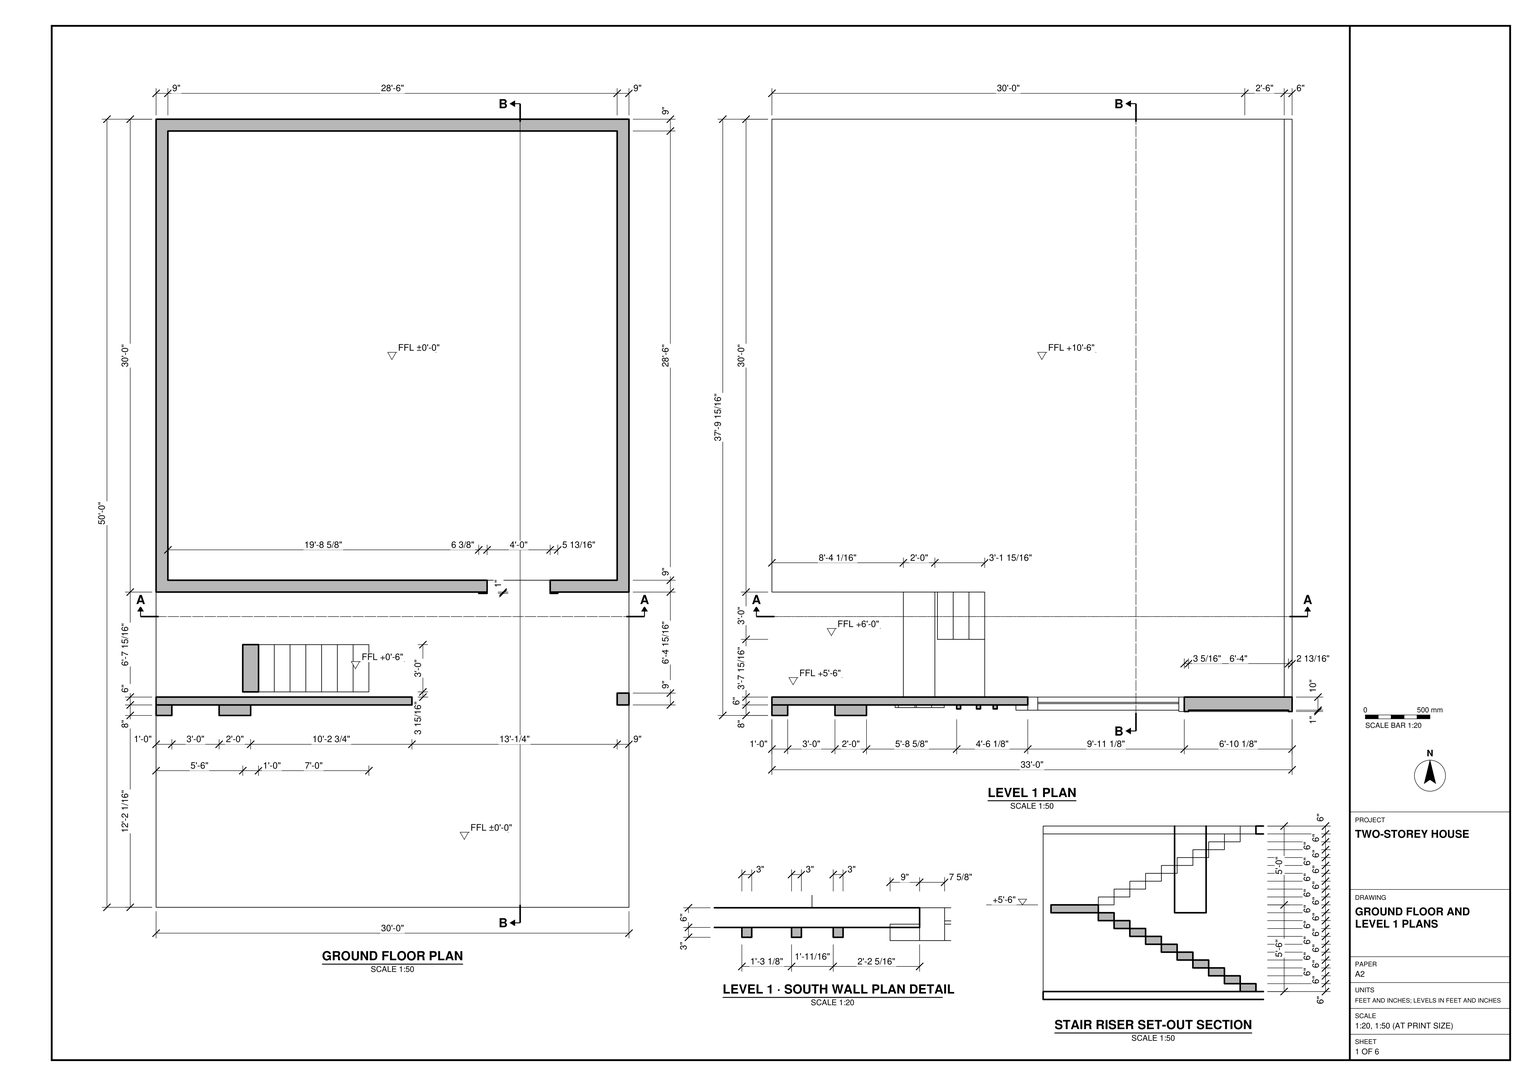
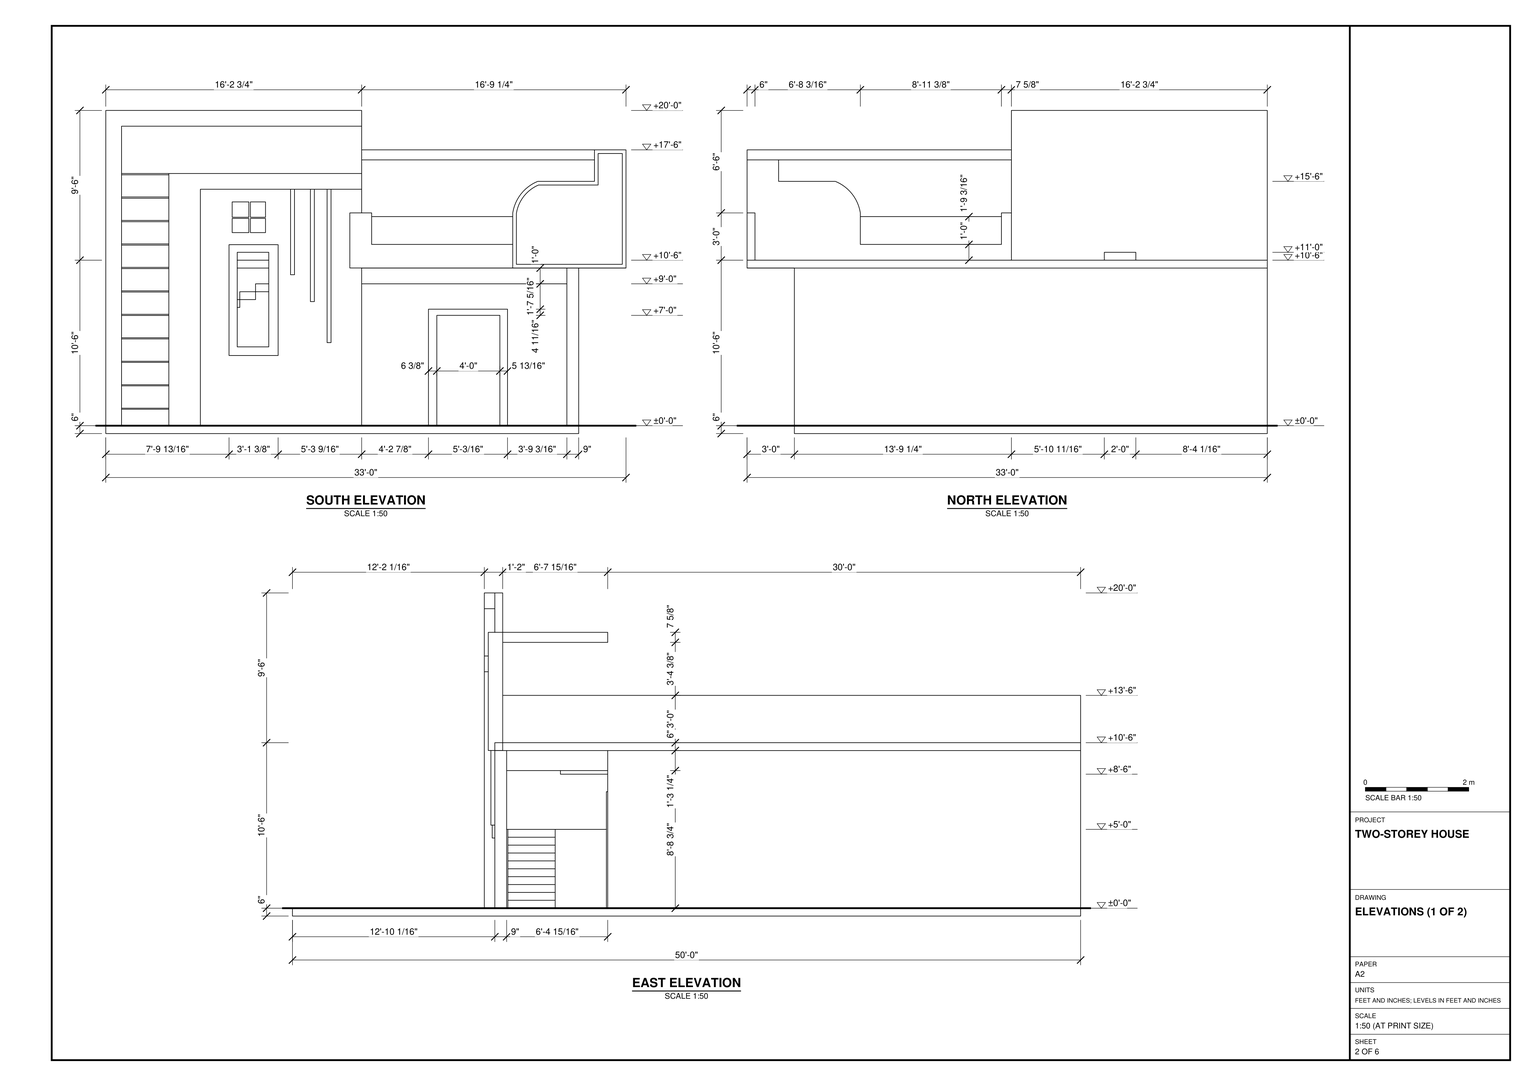
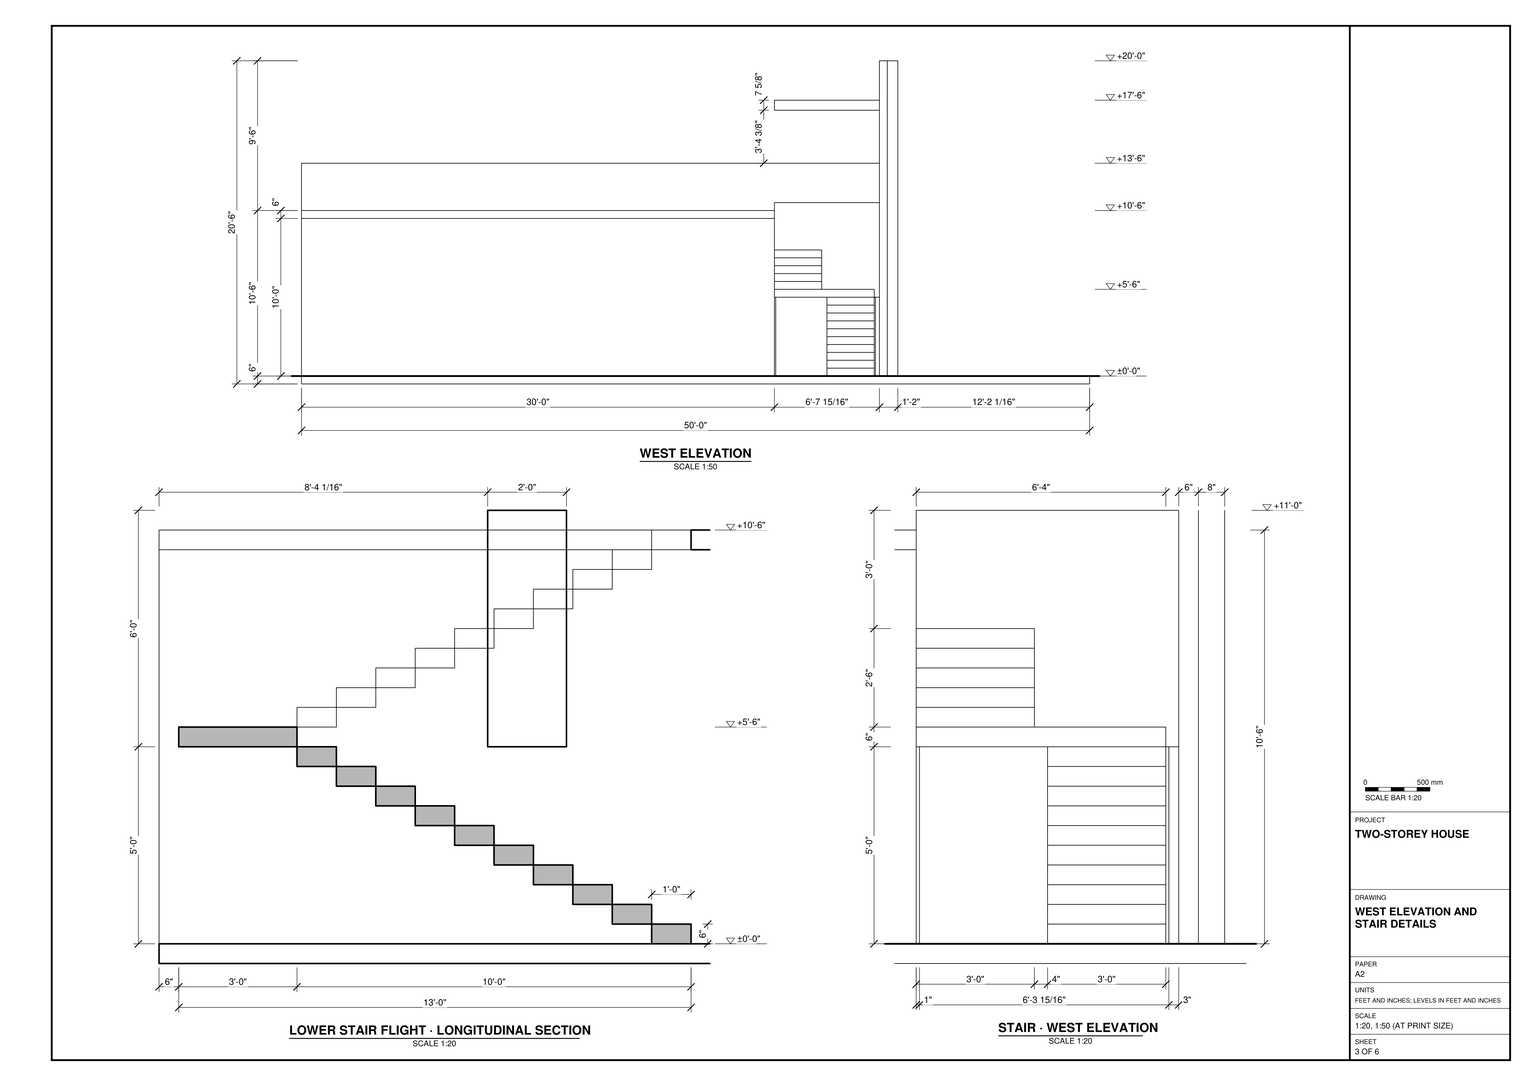
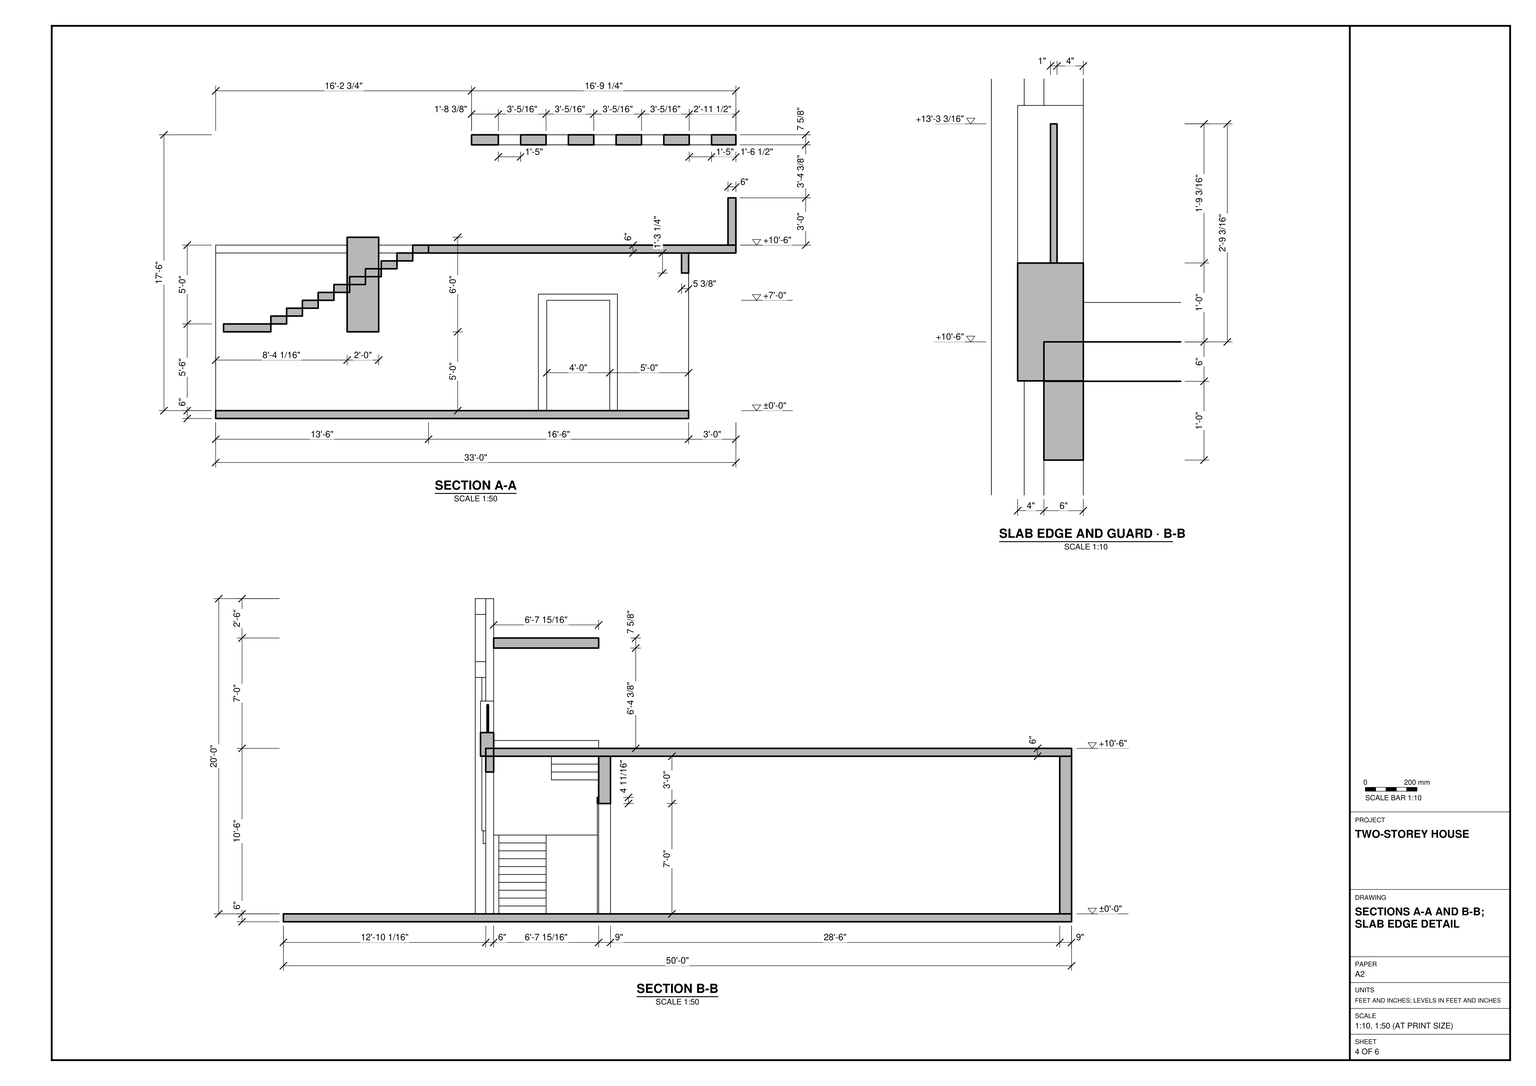
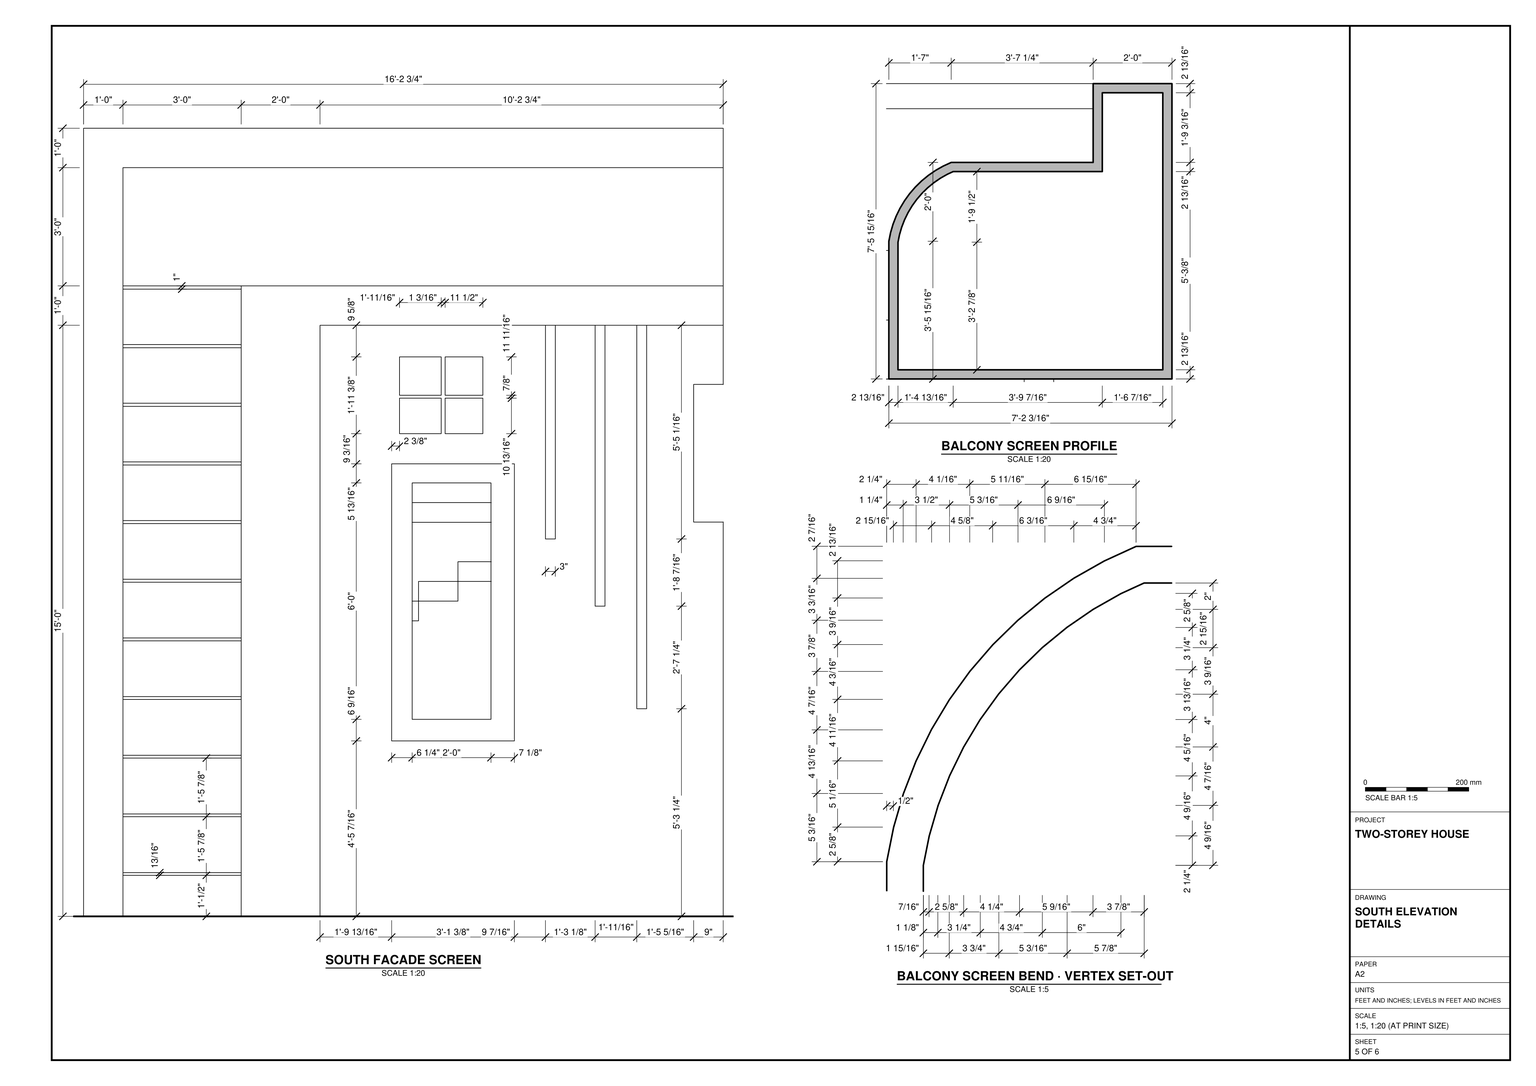
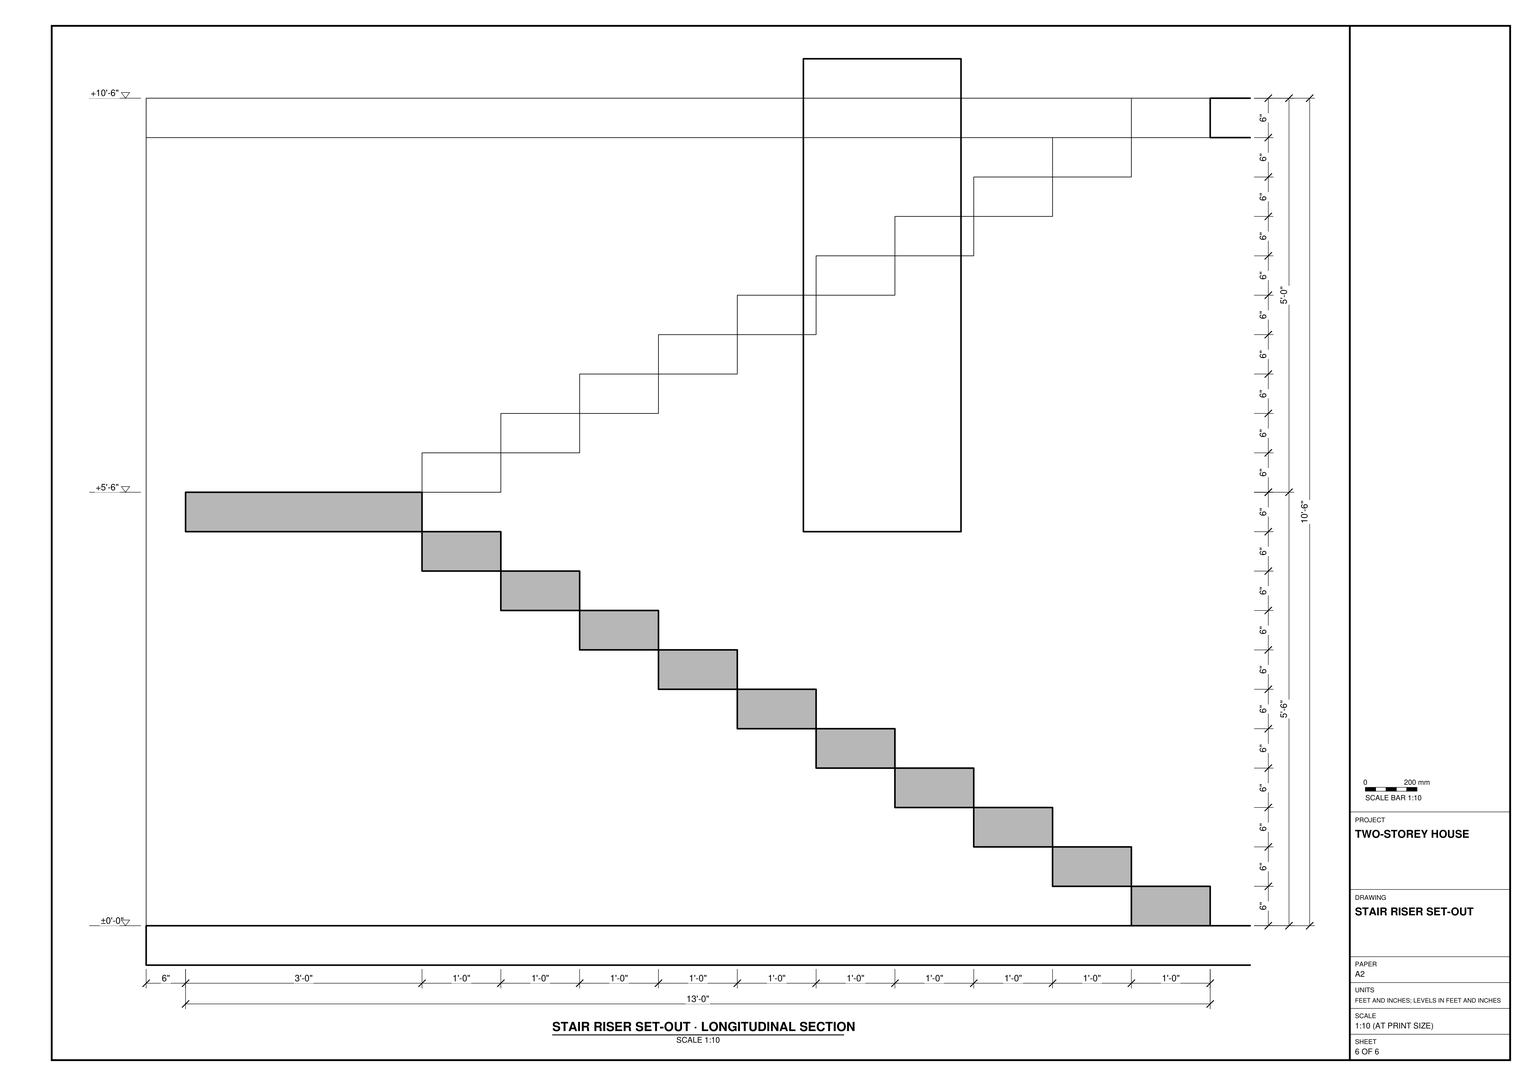
Build the house shown in task_files/diagram_01.pdf in SketchUp. Work in feet and inches. The overall model is 33'-0" wide east to west, 50'-0" deep north to south and 20'-6" high from the underside of the base slab to the top of the south screen. Set the finished floor levels at ±0'-0" and +10'-6".

Place the 30'-0" square ground-floor enclosure at the north end of the base slab. Use the drawn 9" wall thickness and leave the doorway toward the east end of its south wall. Model the flat roof slab as the Level 1 terrace, including its projection beyond the enclosure, its edge walls and the opening for the stair. Between the enclosure and the south screen, model the stair as two parallel flights that reverse direction at the +5'-6" landing. Follow the stair sections for the tread profile and the open space beneath the flights.

Use the elevations to shape the south screen on both sides of the entrance. Include the horizontal divisions at the left, the framed rectangular detail with a divided square above it, the narrow vertical strips and the curved shoulder of the upper panel at the right.

Keep walls, slabs and roof elements in separate groups or components, and do the same for each furniture or joinery piece shown. Use components for repeated parts. Any decor or loose items shown may be represented by suitable library components. Save one SketchUp model as output_files/two_storey_house_with_a_return_stair_and_south_screen.skp.

# SketchUp Ruby script. Lengths in inches.
U = 1.inch
M = Sketchup.active_model
def pt(a) = Geom::Point3d.new(a.map { |v| v * U })
def face(e, loops, mat)
  f = e.add_face(loops[0].map { |a| pt(a) })
  loops[1..].each { |l| e.add_face(l.map { |a| pt(a) }).erase! }
  f.material = f.back_material = mat if mat
  f
end
# faces: each face lists its corners as indices into pts; further lists are holes
def faces(e, pts, list, mat = nil) = list.each { |f| face(e, (f[0].is_a?(Array) ? f : [f]).map { |l| l.map { |i| pts[i] } }, mat) }
# xy, xz, yz: faces in a plane at the given z, y or x. An outline is a flat list of corners, or four numbers for a rectangle; further outlines are holes
def ring(l) = l.size == 4 ? [[l[0], l[1]], [l[2], l[1]], [l[2], l[3]], [l[0], l[3]]] : l.each_slice(2).to_a
def flat(e, list, mat, &to3) = list.each { |f| face(e, (f[0].is_a?(Array) ? f : [f]).map { |l| ring(l).map { |u, v| to3.(u, v) } }, mat) }
def xy(e, z, list, mat = nil) = flat(e, list, mat) { |x, y| [x, y, z] }
def xz(e, y, list, mat = nil) = flat(e, list, mat) { |x, z| [x, y, z] }
def yz(e, x, list, mat = nil) = flat(e, list, mat) { |y, z| [x, y, z] }
def lines(e, pts, list) = list.each { |a, b| e.add_line(pt(pts[a]), pt(pts[b])) }
# prism: a flat outline (further loops are holes) pulled along v
def prism(e, loops, v, mat = nil)
  f = face(e, loops, mat); d = Geom::Vector3d.new(v.map { |x| x * U })
  f.pushpull(f.normal.samedirection?(d) ? d.length : -d.length)
end
def box(e, o, s, mat = nil) = prism(e, [[o, [o[0] + s[0], o[1], o[2]], [o[0] + s[0], o[1] + s[1], o[2]], [o[0], o[1] + s[1], o[2]]]], [0, 0, s[2]], mat)
def at(x, y, z, deg = 0) = Geom::Transformation.translation(pt([x, y, z])) * Geom::Transformation.rotation(ORIGIN, Z_AXIS, deg.degrees)
def axes(o, x, y, z) = Geom::Transformation.new([*x, 0, *y, 0, *z, 0, *pt(o).to_a, 1])
def part(name) = M.definitions.add(name)
# library, detail: a bought-in or finely detailed component or shape, given as its bounding box
def library(name, o, s) = part(name).tap { |d| box(d.entities, o, s) }
def detail(e, o, s) = box(e.add_group.entities, o, s)
def put(e, d, t, mat = nil) = e.add_instance(d, t).tap { |i| i.material = mat if mat }
def group(e, t, mat = nil) = e.add_group.tap { |g| g.transformation = t; g.material = mat if mat }.entities
root = M.entities
M.materials.add("[Formica Blue]").color = [71, 97, 152]
M.materials.add("[Terrazzo Light Blue]").color = [196, 214, 227]
M.materials.add("[Translucent Glass Gray]").color = [128, 128, 128]
M.materials["[Translucent Glass Gray]"].alpha = 0.5
M.materials.add("[Wood OSB]").color = [240, 195, 122]
c1 = part("Stair tread")
box(c1.entities,[0,0,0],[12,36,6])
c2 = part("Stair landing")
box(c2.entities,[0,0,0],[36,76,6])
prism(root,[[[252,240,90],[252,240,6],[245.625,240,6],[245.625,240,94.6875],[305.81,240,94.6875],[305.81,240,6],[300,240,6],[300,240,90]]],[0,-1,0])
xy(root,6,[[0,146.0625,12,154.0625],[48,146.0625,72,154.0625]])
xy(root,59.43,[[93.8125,152.0625,131.1875,154.0625]])
xy(root,66,[[100.0625,152.0625,124.0625,240]])
xy(root,69.23,[[168.46,151.0625,171.46,154.0625]])
xy(root,100.46,[[155.77,151.0625,158.77,154.0625]])
xy(root,120.93,[[140.65,151.0625,143.65,154.0625]])
xy(root,132,[[390,160.0625,396,600]])
xy(root,138,[[100.0625,152.0625,124.0625,240]])
xy(root,143.8,[[93.8125,152.0625,100.0625,154.0625],[100.0625,152.0625,131.1875,154.0625]])
xy(root,144,[[202.39,155.0625,309.79,156.0625]])
xy(root,152.99,[[96.21,152.0625,108.9,154.0625],[110.1,152.0625,121.59,154.0625]])
xy(root,163.8,[[96.21,152.0625,108.9,154.0625],[110.1,152.0625,121.59,154.0625]])
xy(root,164.68,[[96.21,152.0625,108.9,154.0625],[110.1,152.0625,121.59,154.0625]])
xy(root,165.1875,[[202.39,155.0625,309.79,156.0625]],"[Translucent Glass Gray]")
xy(root,168,[[390,160.0625,396,600]])
xy(root,176.37,[[96.21,152.0625,108.9,154.0625],[110.1,152.0625,121.59,154.0625]])
xy(root,186,[[72,146.0625,72,154.0625,140.65,154.0625,140.65,151.0625,143.65,151.0625,143.65,154.0625,155.77,154.0625,155.77,151.0625,158.77,151.0625,158.77,154.0625,168.46,154.0625,168.46,151.0625,171.46,151.0625,171.46,154.0625,194.77,154.0625,194.77,146.0625],[140.65,151.0625,143.65,154.0625],[155.77,151.0625,158.77,154.0625],[168.46,151.0625,171.46,154.0625]])
xy(root,198,[[48,146.0625,194.77,154.0625]],"[Terrazzo Light Blue]")
xy(root,234,[[12,146.0625,194.77,154.0625]])
xy(root,246,[[0,146.0625,194.77,154.0625]])
xz(root,146.0625,[[0,6,12,6,12,234,194.77,234,194.77,246,0,246],[48,6,72,6,72,186,194.77,186,194.77,198,48,198]],"[Terrazzo Light Blue]")
xz(root,151.0625,[[168.46,69.23,171.46,186],[155.77,100.46,158.77,186],[140.65,120.93,143.65,186]],"[Wood OSB]")
xz(root,152.0625,[[[93.8125,59.43,131.1875,143.8],[100.0625,66,124.0625,138]],[96.21,152.99,108.9,163.8],[110.1,152.99,121.59,163.8],[96.21,164.68,108.9,176.37],[110.1,164.68,121.59,176.37]],"[Wood OSB]")
xz(root,154.0625,[[0,6,0,246,194.77,246,194.77,234,12,234,12,6],[48,6,48,198,194.77,198,194.77,186,72,186,72,6],[[93.8125,59.43,131.1875,143.8],[100.0625,66,124.0625,138]],[168.46,69.23,171.46,186],[155.77,100.46,158.77,186],
  [140.65,120.93,143.65,186],[96.21,152.99,108.9,163.8],[110.1,152.99,121.59,163.8],[96.21,164.68,108.9,176.37],[110.1,164.68,121.59,176.37]])
xz(root,155.0625,[[202.39,144,309.79,165.1875]],"[Translucent Glass Gray]")
xz(root,156.0625,[[202.39,144,309.79,165.1875]],"[Translucent Glass Gray]")
xz(root,160.0625,[[390,132,396,168]])
xz(root,240,[[100.0625,66,124.0625,138]])
xz(root,600,[[390,132,396,168]])
yz(root,0,[[146.0625,6,154.0625,246]])
yz(root,12,[[146.0625,6,154.0625,234]],"[Terrazzo Light Blue]")
yz(root,48,[[146.0625,6,154.0625,198]])
yz(root,72,[[146.0625,6,154.0625,186]],"[Terrazzo Light Blue]")
yz(root,93.8125,[[152.0625,59.43,154.0625,143.8]])
yz(root,96.21,[[152.0625,152.99,154.0625,163.8],[152.0625,164.68,154.0625,176.37]])
yz(root,100.0625,[[152.0625,66,240,138]])
yz(root,108.9,[[152.0625,152.99,154.0625,163.8],[152.0625,164.68,154.0625,176.37]])
yz(root,110.1,[[152.0625,152.99,154.0625,163.8],[152.0625,164.68,154.0625,176.37]])
yz(root,121.59,[[152.0625,152.99,154.0625,163.8],[152.0625,164.68,154.0625,176.37]])
yz(root,124.0625,[[152.0625,66,240,138]])
yz(root,131.1875,[[152.0625,59.43,154.0625,143.8]])
yz(root,140.65,[[151.0625,120.93,154.0625,186]])
yz(root,143.65,[[151.0625,120.93,154.0625,186]])
yz(root,155.77,[[151.0625,100.46,154.0625,186]])
yz(root,158.77,[[151.0625,100.46,154.0625,186]])
yz(root,168.46,[[151.0625,69.23,154.0625,186]])
yz(root,171.46,[[151.0625,69.23,154.0625,186]])
yz(root,194.77,[[146.0625,186,154.0625,198],[146.0625,234,154.0625,246]])
yz(root,202.39,[[155.0625,144,156.0625,165.1875]])
yz(root,309.79,[[155.0625,144,156.0625,165.1875]])
yz(root,390,[[160.0625,132,600,168]])
yz(root,396,[[160.0625,132,600,168]],"[Terrazzo Light Blue]")
p = [[12,154.0625,198],[48,154.0625,198],[12,154.0625,180.13],[48,154.0625,180.13],[12,154.0625,162.26],[48,154.0625,162.26],
  [12,154.0625,144.39],[48,154.0625,144.39],[12,154.0625,126.52],[48,154.0625,126.52],[12,154.0625,108.66],[48,154.0625,108.66],
  [12,154.0625,90.79],[48,154.0625,90.79],[12,154.0625,72.92],[48,154.0625,72.92],[12,154.0625,55.05],[48,154.0625,55.05],
  [12,154.0625,37.18],[48,154.0625,37.18],[12,154.0625,19.3125],[48,154.0625,19.3125],[12,154.0625,197],[48,154.0625,197],
  [12,154.0625,179.15],[48,154.0625,179.15],[12,154.0625,161.3],[48,154.0625,161.3],[12,154.0625,143.45],[48,154.0625,143.45],
  [12,154.0625,125.6],[48,154.0625,125.6],[12,154.0625,107.75],[48,154.0625,107.75],[12,154.0625,89.9],[48,154.0625,89.9],
  [12,154.0625,72.05],[48,154.0625,72.05],[12,154.0625,54.2],[48,154.0625,54.2],[12,154.0625,36.35],[48,154.0625,36.35],
  [12,154.0625,18.5],[48,154.0625,18.5]]
lines(root,p,[[0,1],[2,3],[4,5],[6,7],[8,9],[10,11],[12,13],[14,15],[16,17],[18,19],[20,21],[22,23],
  [24,25],[26,27],[28,29],[30,31],[32,33],[34,35],[36,37],[38,39],[40,41],[42,43]])
put(root,c1,at(150,164,6))
put(root,c1,at(138,164,12))
put(root,c1,at(126,164,18))
put(root,c1,at(114,164,24))
put(root,c1,at(102,164,30))
put(root,c1,at(90,164,36))
put(root,c1,at(78,164,42))
put(root,c1,at(66,164,48))
put(root,c1,at(54,164,54))
put(root,c1,at(42,164,60))
put(root,c1,at(54,240,72,180))
put(root,c1,at(78,240,84,180))
put(root,c1,at(162,240,126,180))
put(root,c1,at(126,240,108,180))
put(root,c1,at(66,240,78,180))
put(root,c1,at(150,240,120,180))
put(root,c1,at(90,240,90,180))
put(root,c1,at(102,240,96,180))
put(root,c1,at(114,240,102,180))
put(root,c1,at(138,240,114,180))
put(root,c2,at(6,164,66))
g1 = group(root,at(0,240,0))
box(g1,[0,-240,0],[360,600,6])
g2 = group(root,at(0,240,126))
prism(g2,[[[0,0,0],[0,360,0],[396,360,0],[396,-85.9375,0],[194.77,-85.9375,0],[194.77,-79.9375,0],[162,-79.9375,0],[162,0,0]]],[0,0,6])
g3 = group(root,at(0,240,6),"[Terrazzo Light Blue]")
xy(g3,0,[[0,0,0,360,360,360,360,0,300,0,300,9,351,9,351,351,9,351,9,9,252,9,252,0],[9,9,351,351]])
xy(g3,84,[[252,0,300,9]])
xy(g3,120,[[[0,0,360,360],[9,9,351,351]]])
xz(g3,0,[[0,0,252,0,252,84,300,84,300,0,360,0,360,120,0,120]])
xz(g3,9,[[9,0,9,120,351,120,351,0,300,0,300,84,252,84,252,0]])
xz(g3,351,[[9,0,351,120]])
xz(g3,360,[[0,0,360,120]])
yz(g3,0,[[0,0,360,120]])
yz(g3,9,[[9,0,351,120]])
yz(g3,252,[[0,0,9,84]])
yz(g3,300,[[0,0,9,84]])
yz(g3,351,[[9,0,351,120]])
yz(g3,360,[[0,0,360,120]])
g4 = group(root,at(0,154.0625,6),"[Formica Blue]")
prism(g4,[[[194.77,6,0],[0,6,0],[0,6,240],[194.77,6,240]],[[100.0625,6,60],[124.0625,6,60],[124.0625,6,132],[100.0625,6,132]]],[0,-6,0])
g5 = group(root,at(351,154.0625,6),"[Terrazzo Light Blue]")
box(g5,[0,0,0],[9,9,120])
g6 = group(root,at(194.77,154.0625,114),"[Terrazzo Light Blue]")
box(g6,[0,0,0],[156.23,6,12])
g7 = group(root,at(354.625,163.0625,110.75),"[Terrazzo Light Blue]")
box(g7,[0,0,0],[5.375,76.9375,15.25])
g8 = group(root,at(185.77,150.0625,126.0625),"[Terrazzo Light Blue]")
xy(g8,0,[[124.02,-1,124.02,0,0,0,0,4,9,4,9,10,210.23,10,210.23,-1]])
xy(g8,2.79,[[126.8,-1,207.4375,0]])
xy(g8,17.9375,[[16.61,0,124.02,10]])
xy(g8,41.9375,[[0,0,9,5],[9,0,16.61,10]])
xy(g8,63.15,[[143.6,-1,189.01,0]])
xy(g8,65.9375,[[142.99,-1,186.23,10]])
xy(g8,87.15,[[189.01,-1,207.4375,0]])
xy(g8,89.9375,[[186.23,-1,210.23,10]])
xz(g8,-1,[[[124.02,0,210.23,0,210.23,89.9375,186.23,89.9375,186.23,65.9375,142.99,65.9375,140.57,64.83,138.25,63.51,136.06,62,134,60.3125,132.09,58.45,130.35,56.43,128.79,54.27,127.42,51.99,126.24,49.6,125.28,47.11,124.54,44.55,124.02,41.9375],[126.8,2.79,126.8,41.66,127.25,43.89,127.93,46.22,128.8,48.48,129.87,50.66,131.12,52.74,132.54,54.7,134.12,56.54,135.86,58.23,137.73,59.77,139.73,61.15,141.84,62.34,143.6,63.15,189.01,63.15,189.01,87.15,207.4375,87.15,207.4375,2.79]]],"[Wood OSB]")
xz(g8,0,[[0,0,124.02,0,124.02,17.9375,16.61,17.9375,16.61,41.9375,0,41.9375]])
xz(g8,0,[[126.8,2.79,207.4375,2.79,207.4375,87.15,189.01,87.15,189.01,63.15,143.6,63.15,141.84,62.34,139.73,61.15,137.73,59.77,135.86,58.23,134.12,56.54,132.54,54.7,131.12,52.74,129.87,50.66,128.8,48.48,127.93,46.22,127.25,43.89,126.8,41.66]],"[Formica Blue]")
xz(g8,4,[[0,0,9,5.9375]])
xz(g8,10,[[9,0,9,41.9375,16.61,41.9375,16.61,17.9375,124.02,17.9375,124.02,41.9375,124.54,44.55,125.28,47.11,126.24,49.6,127.42,51.99,128.79,54.27,130.35,56.43,132.09,58.45,134,60.3125,136.06,62,138.25,63.51,140.57,64.83,142.99,65.9375,186.23,65.9375,186.23,89.9375,210.23,89.9375,210.23,0]])
yz(g8,0,[[0,0,0,41.9375,5,41.9375,4,5.9375,4,0]])
yz(g8,9,[[4,0,4,5.9375,5,41.9375,10,41.9375,10,0]])
yz(g8,16.61,[[0,17.9375,10,41.9375]])
yz(g8,124.02,[[-1,0,0,17.9375],[-1,17.9375,10,41.9375]])
yz(g8,126.8,[[-1,2.79,0,17.9375],[-1,17.9375,0,41.66]])
yz(g8,186.23,[[-1,65.9375,10,89.9375]])
yz(g8,189.01,[[-1,63.15,0,87.15]])
yz(g8,207.4375,[[-1,2.79,0,87.15]])
yz(g8,210.23,[[-1,0,10,89.9375]])
p = [[9,5,41.9375],[9,4,5.9375],[0,4,5.9375],[0,5,41.9375],[126.8,0,41.66],[127.25,0,43.89],
  [127.25,-1,43.89],[126.8,-1,41.66],[124.02,10,41.9375],[124.02,-1,41.9375],[124.54,-1,44.55],[124.54,10,44.55],
  [127.93,0,46.22],[127.93,-1,46.22],[125.28,-1,47.11],[125.28,10,47.11],[128.8,0,48.48],[128.8,-1,48.48],
  [126.24,-1,49.6],[126.24,10,49.6],[129.87,0,50.66],[129.87,-1,50.66],[127.42,-1,51.99],[127.42,10,51.99],
  [131.12,0,52.74],[131.12,-1,52.74],[128.79,-1,54.27],[128.79,10,54.27],[132.54,0,54.7],[132.54,-1,54.7],
  [130.35,-1,56.43],[130.35,10,56.43],[134.12,0,56.54],[134.12,-1,56.54],[132.09,-1,58.45],[132.09,10,58.45],
  [135.86,0,58.23],[135.86,-1,58.23],[137.73,0,59.77],[137.73,-1,59.77],[134,-1,60.3125],[134,10,60.3125],
  [139.73,0,61.15],[139.73,-1,61.15],[136.06,-1,62],[136.06,10,62],[141.84,0,62.34],[141.84,-1,62.34],
  [138.25,-1,63.51],[138.25,10,63.51],[143.6,0,63.15],[143.6,-1,63.15],[140.57,-1,64.83],[140.57,10,64.83],
  [142.99,-1,65.9375],[142.99,10,65.9375]]
faces(g8,p,[[0,1,2,3],[4,5,6,7],[8,9,10,11],[5,12,13,6],[11,10,14,15],[12,16,17,13],[15,14,18,19],[16,20,21,17],
  [19,18,22,23],[20,24,25,21],[23,22,26,27],[24,28,29,25],[27,26,30,31],[28,32,33,29],[31,30,34,35],[32,36,37,33],
  [36,38,39,37],[35,34,40,41],[38,42,43,39],[41,40,44,45],[42,46,47,43],[45,44,48,49],[46,50,51,47],[49,48,52,53],
  [53,52,54,55]])
g9 = group(root,at(194.77,160.0625,208.35))
xy(g9,0,[[[0,0,201.23,79.9375],[165.7,15.94,182.7,64.63],[129.37,15.94,146.37,64.63],[93.04,15.94,110.04,64.63],[56.71,15.94,73.71,64.63],[20.39,15.94,37.39,64.63]]])
xy(g9,7.65,[[[0,0,201.23,79.9375],[165.7,15.94,182.7,64.63],[129.37,15.94,146.37,64.63],[93.04,15.94,110.04,64.63],[56.71,15.94,73.71,64.63],[20.39,15.94,37.39,64.63]]],"[Terrazzo Light Blue]")
xz(g9,0,[[0,0,201.23,7.65]],"[Terrazzo Light Blue]")
xz(g9,15.94,[[20.39,0,37.39,7.65],[56.71,0,73.71,7.65],[93.04,0,110.04,7.65],[129.37,0,146.37,7.65],[165.7,0,182.7,7.65]])
xz(g9,64.63,[[20.39,0,37.39,7.65],[56.71,0,73.71,7.65],[129.37,0,146.37,7.65],[165.7,0,182.7,7.65]])
xz(g9,64.63,[[93.04,0,110.04,7.65]],"[Terrazzo Light Blue]")
xz(g9,79.9375,[[0,0,201.23,7.65]])
yz(g9,0,[[0,0,79.9375,7.65]])
yz(g9,20.39,[[15.94,0,64.63,7.65]])
yz(g9,37.39,[[15.94,0,64.63,7.65]])
yz(g9,56.71,[[15.94,0,64.63,7.65]])
yz(g9,73.71,[[15.94,0,64.63,7.65]])
yz(g9,93.04,[[15.94,0,64.63,7.65]],"[Terrazzo Light Blue]")
yz(g9,110.04,[[15.94,0,64.63,7.65]])
yz(g9,129.37,[[15.94,0,64.63,7.65]])
yz(g9,146.37,[[15.94,0,64.63,7.65]])
yz(g9,165.7,[[15.94,0,64.63,7.65]])
yz(g9,182.7,[[15.94,0,64.63,7.65]])
yz(g9,201.23,[[0,0,79.9375,7.65]])
